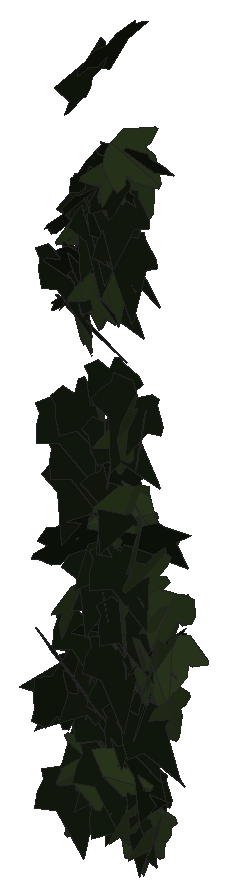
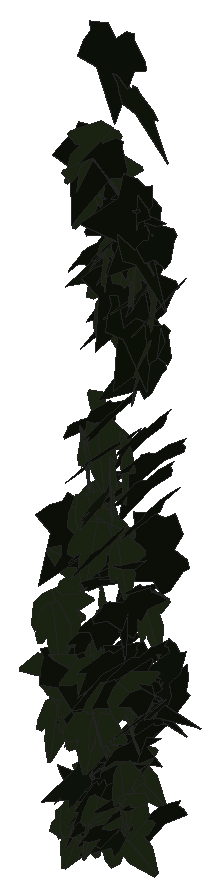
# SketchUp Ruby script. Lengths in inches.
U = 1.inch
M = Sketchup.active_model
def pt(a) = Geom::Point3d.new(a.map { |v| v * U })
def face(e, loops, mat)
  f = e.add_face(loops[0].map { |a| pt(a) })
  loops[1..].each { |l| e.add_face(l.map { |a| pt(a) }).erase! }
  f.material = f.back_material = mat if mat
  f
end
# faces: each face lists its corners as indices into pts; further lists are holes
def faces(e, pts, list, mat = nil) = list.each { |f| face(e, (f[0].is_a?(Array) ? f : [f]).map { |l| l.map { |i| pts[i] } }, mat) }
# xy, xz, yz: faces in a plane at the given z, y or x. An outline is a flat list of corners, or four numbers for a rectangle; further outlines are holes
def ring(l) = l.size == 4 ? [[l[0], l[1]], [l[2], l[1]], [l[2], l[3]], [l[0], l[3]]] : l.each_slice(2).to_a
def flat(e, list, mat, &to3) = list.each { |f| face(e, (f[0].is_a?(Array) ? f : [f]).map { |l| ring(l).map { |u, v| to3.(u, v) } }, mat) }
def xy(e, z, list, mat = nil) = flat(e, list, mat) { |x, y| [x, y, z] }
def xz(e, y, list, mat = nil) = flat(e, list, mat) { |x, z| [x, y, z] }
def yz(e, x, list, mat = nil) = flat(e, list, mat) { |y, z| [x, y, z] }
def lines(e, pts, list) = list.each { |a, b| e.add_line(pt(pts[a]), pt(pts[b])) }
# prism: a flat outline (further loops are holes) pulled along v
def prism(e, loops, v, mat = nil)
  f = face(e, loops, mat); d = Geom::Vector3d.new(v.map { |x| x * U })
  f.pushpull(f.normal.samedirection?(d) ? d.length : -d.length)
end
def box(e, o, s, mat = nil) = prism(e, [[o, [o[0] + s[0], o[1], o[2]], [o[0] + s[0], o[1] + s[1], o[2]], [o[0], o[1] + s[1], o[2]]]], [0, 0, s[2]], mat)
def at(x, y, z, deg = 0) = Geom::Transformation.translation(pt([x, y, z])) * Geom::Transformation.rotation(ORIGIN, Z_AXIS, deg.degrees)
def axes(o, x, y, z) = Geom::Transformation.new([*x, 0, *y, 0, *z, 0, *pt(o).to_a, 1])
def part(name) = M.definitions.add(name)
# library, detail: a bought-in or finely detailed component or shape, given as its bounding box
def library(name, o, s) = part(name).tap { |d| box(d.entities, o, s) }
def detail(e, o, s) = box(e.add_group.entities, o, s)
def put(e, d, t, mat = nil) = e.add_instance(d, t).tap { |i| i.material = mat if mat }
def group(e, t, mat = nil) = e.add_group.tap { |g| g.transformation = t; g.material = mat if mat }.entities
root = M.entities
M.materials.add("efeu1").color = [18, 25, 13]
M.materials.add("efeu2").color = [43, 57, 29]
c1 = part("ivyleaf_10")
p = [[0,0.5,-0.03],[-0.0625,2.02,-0.43],[-0.19,2.01,-0.46],[-0.54,1.05,-0.29],[-0.52,0.625,-0.18],[-0.83,0.76,-0.28],
  [-1.16,0.64,-0.33],[-1.15,0.33,-0.24],[-0.77,-0.39,0.02],[-0.3,-0.51,0.16],[0.04,-0.48,0.23],[-0.02,2.01,-0.4375],
  [-0.06,2.01,-0.43],[0.04,-0.49,0.23],[0.67,-0.49,0.14],[1.38,0.36,-0.2],[1.375,0.51,-0.24],[0.81,0.65,-0.19],
  [0.62,0.59,-0.15],[0.6,1.09,-0.28],[0.5,1.23,-0.31]]
faces(c1.entities,p,[[0,1,2,3,4,5,6,7,8,9,10],[11,12,0,13,14,15,16,17,18,19,20]],"efeu2")
c2 = part("ivyleaf_9")
p = [[1.54,2.16,1.25],[1.36,2.04,1.19],[-0.21,0.99,0.68],[-0.71,1.11,0.82],[-0.85,0.86,0.67],[-0.8,0.17,0.21],
  [-0.9,-0.01,0.1],[-0.67,-0.16,-0.02],[-0.08,-0.08,-0.05],[-0.03,-0.6,-0.4],[0.65,-0.88,-0.66],[0.83,-0.6,-0.49],
  [1.29,-0.42,-0.43],[1.8125,-0.07,-0.26],[1.21,0.44,0.15]]
faces(c2.entities,p,[[0,1,2,3,4,5,6,7,8,9,10,11,12,13,14]],"efeu1")
put(root,c1,axes([520.53,134.19,209.15],[0.11918,-0.84197,-0.10734],[0.00558,0.10917,-0.85011],[0.84877,0.1175,0.02066]))
put(root,c2,axes([520.25,134.12,210.57],[-0.08598,-0.85654,0.06344],[-0.00408,-0.06335,-0.86085],[0.85888,-0.08604,0.00226]))
put(root,c2,axes([520.21,133.12,207.36],[-0.08395,-0.8203,-0.28988],[0.07021,0.28389,-0.82368],[0.86717,-0.1024,0.03862]))
put(root,c1,axes([520.52,133.03,225.07],[-0.47607,0.77088,0.19871],[-0.10838,0.16662,-0.90603],[-0.78867,-0.48823,0.00456]))
put(root,c1,axes([520.63,133.88,212.37],[-0.31595,-0.54289,0.58824],[-0.02392,-0.62572,-0.59033],[0.80012,-0.23308,0.21463]))
put(root,c2,axes([521.2,133.08,211.59],[-0.74159,0.06419,0.53106],[-0.52862,0.05109,-0.74435],[-0.08192,-0.9107,-0.00433]))
put(root,c1,axes([520.16,133.93,207.99],[0.11338,-0.19335,-0.83228],[0.54128,0.66588,-0.08095],[0.66113,-0.51201,0.20901]))
put(root,c2,axes([520.08,132.67,226.9375],[0.40949,-0.84435,-0.11484],[0.00597,0.13025,-0.93637],[0.8521,0.40485,0.06175]))
put(root,c2,axes([520.15,132.92,221.24],[0.12492,-0.82781,-0.32581],[0.09883,0.33988,-0.82567],[0.88411,0.07897,0.13833]))
put(root,c2,axes([520.66,132.73,225.875],[0.38716,0.78249,0.28941],[-0.00289,0.32032,-0.86217],[-0.8343,0.36201,0.13729]))
put(root,c2,axes([520.09,133.07,225.01],[0.88292,-0.25971,0.02898],[0.04536,0.05178,-0.9182],[0.25735,0.88188,0.06244]))
put(root,c2,axes([520.17,133.56,211.38],[0.51099,-0.59355,-0.38575],[-0.00782,0.47099,-0.73507],[0.70785,0.43368,0.27035]))
put(root,c2,axes([520.49,134.2,215.93],[-0.30685,-0.80497,-0.14554],[0.02294,0.14692,-0.86094],[0.8177,-0.3062,-0.03046]))
put(root,c2,axes([520.61,131.89,210.63],[-0.23596,-0.3809,0.88967],[0.54905,0.7014,0.44591],[-0.79695,0.596,0.0438]))
put(root,c2,axes([519.93,132.55,212.32],[0.63136,-0.60151,0.43671],[0.31249,-0.30511,-0.87201],[0.67445,0.70445,-0.00478]))
put(root,c1,axes([521.15,133.51,206.48],[-0.49098,-0.35359,0.63048],[-0.53014,-0.34199,-0.60464],[0.49141,-0.72222,-0.02236]))
put(root,c2,axes([521.03,132.97,226.43],[-0.21695,0.90548,-0.00616],[0.01348,-0.00311,-0.93102],[-0.9054,-0.21702,-0.01238]))
put(root,c2,axes([520.3,134.05,208.78],[0.49852,-0.68551,-0.13966],[-0.06103,0.12822,-0.84723],[0.69693,0.50158,0.0257]))
put(root,c1,axes([520.8125,132.55,214.86],[0.1681,-0.85845,0.10884],[0.00555,-0.10981,-0.87461],[0.8653,0.16747,-0.01554]))
put(root,c2,axes([520.3125,133.4,211.53],[0.47929,-0.75573,-0.05224],[-0.02141,0.04828,-0.89487],[0.75723,0.4797,0.00777]))
put(root,c1,axes([520.62,132.58,227.17],[-0.66362,0.59101,-0.30182],[0.15772,-0.27414,-0.8836],[-0.6446,-0.67552,0.09452]))
put(root,c2,axes([521.25,132.71,229.18],[-0.52731,0.77765,-0.02322],[0.01175,-0.02009,-0.93957],[-0.77791,-0.52744,0.00155]))
put(root,c2,axes([520.5,133.35,213.4],[0.10648,-0.83522,-0.26526],[0.01115,0.26848,-0.84088],[0.87626,0.09808,0.04293]))
put(root,c2,axes([520.58,133.0625,218.68],[-0.11408,-0.81287,0.38841],[0.0355,-0.39526,-0.81679],[0.9002,-0.08743,0.08144]))
put(root,c1,axes([520.56,133.73,211.16],[0.46858,-0.4986,0.5259],[0.37404,-0.36999,-0.68406],[0.62069,0.59937,0.01521]))
put(root,c2,axes([520.49,131.7,216.875],[0.56801,0.40342,0.70098],[0.52261,0.47066,-0.69434],[-0.61725,0.76973,0.05718]))
put(root,c2,axes([520.54,132.93,220.05],[0.23784,-0.82499,-0.31362],[-0.0134,0.32139,-0.85561],[0.88249,0.22723,0.07153]))
put(root,c2,axes([520.6875,134.91,207.65],[-0.04769,-0.83724,-0.05007],[-0.0029,0.05031,-0.83858],[0.83873,-0.04743,-0.00574]))
put(root,c2,axes([520.53,133.18,212.66],[0.64931,0.38049,0.49242],[0.40521,0.2816,-0.75191],[-0.47229,0.76471,0.03188]))
put(root,c1,axes([521.06,133.64,217.4],[0.07663,-0.8776,-0.04927],[-0.00653,0.04889,-0.88093],[0.87895,0.07688,-0.00225]))
put(root,c2,axes([521.14,133.87,210.03],[-0.6179,-0.57593,0.17462],[-0.09895,-0.14963,-0.84369],[0.59363,-0.62442,0.04112]))
put(root,c1,axes([521.61,132.8,208.73],[-0.51218,-0.28882,0.75947],[-0.6743,-0.34982,-0.58778],[0.45335,-0.84661,-0.01622]))
put(root,c2,axes([521.46,132.79,211.64],[-0.91078,-0.05074,0.10069],[-0.10033,-0.00921,-0.91218],[0.05144,-0.91628,0.00359]))
put(root,c2,axes([520.64,132.8,221.95],[0.37772,-0.72988,-0.37118],[-0.06321,0.38156,-0.81461],[0.8164,0.36723,0.10866]))
put(root,c2,axes([521.62,132.29,234.38],[-0.54051,0.74449,0.27635],[-0.18369,0.20802,-0.91966],[-0.77259,-0.57031,0.02531]))
put(root,c2,axes([520.97,131.85,229.3],[0.39321,0.67448,0.53432],[0.20374,0.49778,-0.77829],[-0.83601,0.43855,0.06164]))
put(root,c2,axes([521.6,132.85,215.29],[0.0944,0.21642,-0.88082],[-0.8901,0.19234,-0.04814],[0.17436,0.86473,0.23115]))
put(root,c1,axes([521.23,132.73,227.31],[0.43768,-0.74713,-0.32841],[0.03491,0.38946,-0.83948],[0.81537,0.38437,0.21223]))
put(root,c2,axes([520.88,134.31,213.83],[0.21325,-0.71466,-0.43865],[0.02556,0.45794,-0.73367],[0.83816,0.16787,0.13398]))
put(root,c1,axes([521.21,133.92,211.94],[-0.29662,-0.7641,-0.46343],[0.22526,0.4086,-0.81787],[0.8648,-0.36851,0.05409]))
put(root,c2,axes([521.12,133.72,215.52],[-0.2439,-0.85401,0.12371],[-0.00689,-0.12663,-0.88772],[0.8629,-0.2424,0.02788]))
put(root,c2,axes([520.82,133.7,207.27],[0.78074,-0.38751,0.00067],[0.00077,0.00004,-0.87162],[0.38751,0.78074,0.00038]))
put(root,c1,axes([521.375,134.7,211.16],[-0.73054,-0.429,-0.07664],[0.05961,0.04982,-0.84709],[0.4317,-0.73285,-0.01272]))
put(root,c2,axes([521.1,132.6,229.9],[0.17306,0.23053,0.90145],[0.53851,0.72292,-0.28826],[-0.75879,0.56564,0.00102]))
put(root,c1,axes([521.39,134.52,207.79],[-0.02415,-0.69176,-0.48275],[0.04146,0.48139,-0.69188],[0.84253,-0.04352,0.02021]))
put(root,c1,axes([521.38,132.81,227.64],[-0.68707,0.63251,0.03574],[-0.07167,-0.02522,-0.93148],[-0.62946,-0.68754,0.06705]))
put(root,c1,axes([521.38,133.09,221.1],[0.65706,-0.55162,-0.29941],[-0.06218,0.37413,-0.82573],[0.62455,0.61758,0.23279]))
put(root,c2,axes([521.43,132.84,227.29],[0.34437,0.81979,0.29721],[0.02495,0.31016,-0.8844],[-0.87164,0.33276,0.09211]))
put(root,c2,axes([520.87,131.94,227.46],[0.89051,0.2495,0.27417],[0.25351,0.11062,-0.92408],[-0.27046,0.92517,0.03655]))
put(root,c2,axes([520.9375,132.52,227.53],[0.67123,-0.64743,-0.0718],[-0.05189,0.04962,-0.93258],[0.64933,0.67323,-0.00031]))
put(root,c2,axes([521.56,134.04,216.52],[-0.53647,-0.61708,0.31627],[-0.07859,-0.34318,-0.80291],[0.68894,-0.51966,0.15468]))
put(root,c1,axes([521.55,132.47,228.84],[-0.59831,-0.67527,-0.26229],[0.14791,0.21914,-0.90158],[0.70916,-0.61542,-0.03325]))
put(root,c2,axes([521.15,133.44,210.27],[0.19868,-0.79225,-0.3372],[0.0521,0.35649,-0.80687],[0.85944,0.16154,0.12686]))
put(root,c1,axes([521.46,132.72,228.3],[0.92081,-0.16105,-0.05798],[-0.01574,0.23625,-0.90616],[0.17044,0.89187,0.22957]))
put(root,c2,axes([521.33,133.69,214.97],[-0.11091,-0.78383,-0.37772],[0.07349,0.37097,-0.79141],[0.86698,-0.13172,0.01876]))
put(root,c1,axes([521.71,133.28,220.18],[0.46091,-0.62283,-0.4477],[-0.11033,0.46305,-0.75776],[0.75907,0.44549,0.16171]))
put(root,c2,axes([521.72,133.76,208.59],[-0.53715,-0.60991,0.24873],[-0.07995,-0.2582,-0.8058],[0.6538,-0.53266,0.10581]))
put(root,c1,axes([521.94,134.53,210.83],[0.57382,0.24443,-0.58515],[-0.56275,-0.16753,-0.62182],[-0.29234,0.80225,0.04844]))
put(root,c1,axes([521.59,134.33,211.29],[0.48046,-0.69593,0.14974],[0.09501,-0.11635,-0.84559],[0.70549,0.48962,0.0119]))
put(root,c2,axes([521.24,133.05,226.7],[0.43177,-0.70131,-0.42947],[-0.01179,0.47974,-0.79525],[0.82228,0.37513,0.21411]))
put(root,c1,axes([521.85,133.05,226.52],[-0.19599,-0.89751,0.1172],[0.00177,-0.12029,-0.91825],[0.90512,-0.1941,0.02717]))
put(root,c2,axes([521.63,134.41,207.36],[-0.25178,-0.78578,0.22303],[-0.03203,-0.22371,-0.82432],[0.81619,-0.25118,0.03646]))
put(root,c2,axes([522.04,132.6,230.32],[0.56781,0.30967,-0.69401],[-0.6108,-0.32952,-0.64676],[-0.45219,0.83395,0.00215]))
put(root,c2,axes([521.41,133.62,222.72],[0.34596,-0.81009,-0.20481],[-0.00376,0.22016,-0.87716],[0.83557,0.3364,0.08085]))
put(root,c2,axes([521.96,132.84,229.59],[-0.602,-0.70882,-0.12277],[0.10519,0.07163,-0.92936],[0.71165,-0.6102,0.03351]))
put(root,c1,axes([522.22,133.14,212.08],[0.55828,-0.45123,-0.54294],[-0.24054,0.5292,-0.68714],[0.66373,0.57132,0.20766]))
put(root,c2,axes([521.86,133.91,208.16],[0.36219,-0.5327,-0.55435],[-0.31864,0.45366,-0.64413],[0.69967,0.48236,-0.00639]))
put(root,c1,axes([522.09,132.9,228.04],[0.21113,-0.85345,-0.31342],[0.02915,0.32795,-0.87338],[0.90871,0.18777,0.10084]))
put(root,c2,axes([521.6,133.84,219.5],[0.48699,-0.74696,0.00794],[0.04393,0.01918,-0.89043],[0.7457,0.48668,0.04728]))
put(root,c2,axes([521.61,134.77,209.16],[0.66514,-0.52089,0.04945],[0.08819,0.03278,-0.84103],[0.51574,0.66617,0.08005]))
put(root,c2,axes([521.87,132.75,228.94],[0.03811,-0.92513,0.18372],[0.00641,-0.18361,-0.92592],[0.94318,0.03863,-0.00113]))
put(root,c1,axes([522.14,133.88,212.87],[0.26697,0.83917,-0.04994],[-0.121,-0.01349,-0.87359],[-0.83191,0.27127,0.11103]))
put(root,c2,axes([521.74,133.12,221.125],[0.45335,-0.68545,-0.36424],[0.06105,0.452,-0.77461],[0.77381,0.36592,0.27451]))
put(root,c1,axes([522.23,132.3,227.06],[-0.53747,-0.74461,-0.18774],[0.17318,0.10572,-0.91509],[0.74813,-0.55942,0.07696]))
put(root,c2,axes([522,132.86,209.01],[-0.0704,-0.82612,-0.27403],[0.00361,0.27465,-0.8289],[0.87038,-0.06795,-0.01873]))
put(root,c2,axes([522.52,132.11,235.98],[-0.01812,0.96729,0.05748],[0.00049,0.0575,-0.96746],[-0.969,-0.01806,-0.00157]))
put(root,c2,axes([522.8,132.42,231.04],[-0.85712,0.41957,0.01544],[-0.00924,0.01625,-0.95424],[-0.41975,-0.8571,-0.01053]))
put(root,c1,axes([522.42,133.12,221.18],[-0.22477,-0.8951,-0.03345],[-0.00341,0.03534,-0.92281],[0.89572,-0.22448,-0.01191]))
put(root,c2,axes([521.83,132.9375,229.1],[0.43038,-0.82834,0.03911],[0.03696,-0.02486,-0.93323],[0.82843,0.43144,0.02132]))
put(root,c1,axes([522.35,133.42,217.54],[-0.36898,-0.77074,-0.26118],[0.11196,0.23596,-0.85451],[0.80606,-0.38559,-0.00087]))
put(root,c2,axes([521.98,133.54,217.22],[0.25413,-0.85833,-0.13459],[-0.01214,0.13671,-0.89476],[0.86874,0.253,0.02687]))
put(root,c1,axes([522.97,133.27,218.125],[-0.27286,-0.03752,0.86368],[-0.68832,-0.53851,-0.24086],[0.52302,-0.72828,0.1336]))
put(root,c2,axes([521.7,133.57,206.95],[0.13647,-0.20872,0.88748],[0.75131,-0.48258,-0.22903],[0.51645,0.75721,0.09866]))
put(root,c2,axes([522.21,133.24,218.74],[-0.21864,-0.79777,0.37994],[0.05427,-0.40278,-0.81451],[0.88196,-0.17299,0.1443]))
put(root,c1,axes([521.82,132.3,208.58],[-0.14344,-0.23425,-0.87554],[0.85468,0.26004,-0.2096],[0.30163,-0.84825,0.17753]))
put(root,c2,axes([522.16,132.9375,212.85],[0.09657,-0.89431,-0.03993],[-0.0056,0.03956,-0.89951],[0.89518,0.09673,-0.00132]))
put(root,c2,axes([522.14,133.43,214.28],[0.20962,-0.78359,-0.36918],[-0.03957,0.37077,-0.80945],[0.8653,0.20678,0.05241]))
put(root,c2,axes([522.17,133.1,211.3],[0.09153,-0.87935,0.08662],[-0.00292,-0.08739,-0.88402],[0.8836,0.0908,-0.0119]))
put(root,c2,axes([521.98,132.89,228.23],[0.6622,-0.66097,-0.01558],[0.08993,0.11189,-0.92467],[0.65501,0.65286,0.14271]))
put(root,c2,axes([522.45,132.53,230],[-0.65371,-0.51874,-0.45344],[0.36588,0.26827,-0.83439],[0.58381,-0.74899,0.01519]))
put(root,c1,axes([522.74,132.55,231.17],[-0.49041,-0.77907,0.21994],[-0.03957,-0.23378,-0.9163],[0.80856,-0.48396,0.08856]))
put(root,c1,axes([522.68,133,218.81],[-0.25978,-0.83661,0.22386],[0.03278,-0.24305,-0.87027],[0.86542,-0.24192,0.10016]))
put(root,c1,axes([522.47,134.17,211.73],[-0.82582,-0.0913,-0.2792],[0.29211,-0.1675,-0.80924],[0.03094,-0.85549,0.18825]))
put(root,c2,axes([522.49,133.57,222.11],[-0.29721,-0.83427,0.17684],[0.00217,-0.18801,-0.88333],[0.85281,-0.29027,0.06388]))
put(root,c1,axes([522.61,133.68,221.28],[0.59901,-0.66904,-0.05326],[0.05072,0.11631,-0.89059],[0.66923,0.59002,0.11517]))
put(root,c2,axes([522.27,133.03,207.45],[0.00438,-0.65503,-0.56743],[0.20172,0.55262,-0.63638],[0.84283,-0.12886,0.15526]))
put(root,c2,axes([522.78,133.26,209.8],[0.14105,-0.01041,0.9238],[0.11896,0.92693,-0.00772],[-0.91617,0.11876,0.14122]))
put(root,c1,axes([522.99,133.54,206.72],[-0.61314,-0.45216,0.3727],[-0.26437,-0.26795,-0.76],[0.52294,-0.66562,0.05277]))
put(root,c1,axes([522.5,133.34,212.92],[-0.71339,0.34867,-0.38991],[0.28356,-0.2963,-0.78378],[-0.43953,-0.75707,0.12719]))
put(root,c1,axes([522.65,133.72,206.52],[-0.67838,-0.4395,-0.24822],[0.21238,0.12868,-0.80828],[0.45789,-0.71082,0.00715]))
put(root,c1,axes([522.39,133,214.71],[-0.31377,0.42234,-0.76207],[0.34151,-0.68555,-0.52054],[-0.80156,-0.45741,0.07653]))
put(root,c1,axes([523.02,132.36,221.53],[0.00582,0.13355,0.92122],[-0.5314,0.75685,-0.10636],[-0.76427,-0.52523,0.08097]))
put(root,c2,axes([523.0625,134.04,212.81],[-0.18416,0.84553,-0.17008],[-0.01211,-0.17643,-0.864],[-0.86239,-0.17808,0.04845]))
put(root,c1,axes([522.875,133.8125,207.1],[-0.10314,-0.82055,0.20963],[0.01989,-0.21347,-0.82578],[0.84667,-0.09494,0.04494]))
put(root,c2,axes([522.51,132.79,216.72],[0.03813,-0.77738,-0.44687],[0.02369,0.44799,-0.77731],[0.89635,0.02123,0.03955]))
put(root,c2,axes([522.59,134.07,208.07],[-0.18965,-0.74936,0.37902],[0.10939,-0.4073,-0.75053],[0.8326,-0.11718,0.18494]))
put(root,c2,axes([522.92,132.44,231.95],[0.76626,0.46985,-0.32593],[-0.35846,-0.02992,-0.88587],[-0.44553,0.83216,0.15218]))
put(root,c2,axes([522.625,133.57,207.05],[0.10932,-0.80647,0.18433],[0.00903,-0.18476,-0.8137],[0.82722,0.1086,-0.01548]))
put(root,c1,axes([522.8,132.5,230.85],[0.47841,0.61423,0.55019],[0.02612,0.62447,-0.71988],[-0.8242,0.37633,0.29655]))
put(root,c2,axes([522.74,132.97,210.93],[0.19362,-0.73156,-0.43374],[-0.06709,0.43031,-0.75573],[0.84783,0.20112,0.03925]))
put(root,c2,axes([522.75,132.78,228.44],[0.09935,-0.92979,0.03741],[0.00261,-0.03734,-0.93509],[0.93054,0.09938,-0.00137]))
put(root,c1,axes([523.23,132.53,207.55],[0.05355,-0.84845,-0.27109],[-0.01402,0.27074,-0.85013],[0.89059,0.05528,0.00291]))
put(root,c2,axes([522.83,133.84,208.2],[0.02622,-0.6379,0.56107],[0.08916,-0.55617,-0.6365],[0.84485,0.07849,0.04976]))
put(root,c1,axes([523.42,132.72,212.81],[0.49038,-0.52338,-0.51154],[-0.17086,0.51686,-0.69263],[0.71162,0.48477,0.1862]))
put(root,c1,axes([523.03,132.18,232.14],[0.16039,0.69781,0.63691],[0.14761,0.61958,-0.716],[-0.93317,0.21795,-0.00379]))
put(root,c1,axes([523.3125,132.56,217.72],[0.47656,-0.74407,-0.15768],[-0.01617,0.17612,-0.87996],[0.76042,0.47005,0.08011]))
put(root,c1,axes([523.14,132.98,215.73],[0.06924,-0.66748,0.6504],[0.03552,0.65361,0.66699],[-0.93128,-0.0247,0.07379]))
put(root,c1,axes([523.38,134.15,210.77],[-0.15782,-0.79398,-0.29062],[0.07533,0.28126,-0.80931],[0.84213,-0.17395,0.01793]))
put(root,c1,axes([523.15,133.86,212.3],[0.06729,-0.75129,-0.46612],[0.1244,-0.45478,0.75096],[-0.87534,-0.12238,0.07089]))
put(root,c1,axes([523.25,134.46,212.77],[0.71917,0.48149,-0.00307],[-0.02639,0.03389,-0.86441],[-0.48078,0.71838,0.04284]))
put(root,c2,axes([523.19,133,217.6],[0.71424,0.53164,0.03839],[0.02531,0.03029,-0.89033],[-0.53242,0.71463,0.00918]))
put(root,c1,axes([523.5,134.17,214.37],[-0.14387,-0.86299,-0.03822],[-0.01081,0.04054,-0.87473],[0.86377,-0.14323,-0.01732]))
put(root,c2,axes([523.1,133.0625,210.73],[0.37806,-0.64055,-0.45637],[-0.12154,0.45269,-0.73607],[0.77705,0.38245,0.10691]))
put(root,c1,axes([523.63,133.96,214.77],[-0.53467,-0.62299,0.31586],[-0.10351,-0.32271,-0.81173],[0.69077,-0.53056,0.12284]))
put(root,c1,axes([523.51,133.13,206.55],[0.14346,-0.84014,-0.04863],[-0.01313,0.04709,-0.85228],[0.84144,0.14397,-0.00501]))
